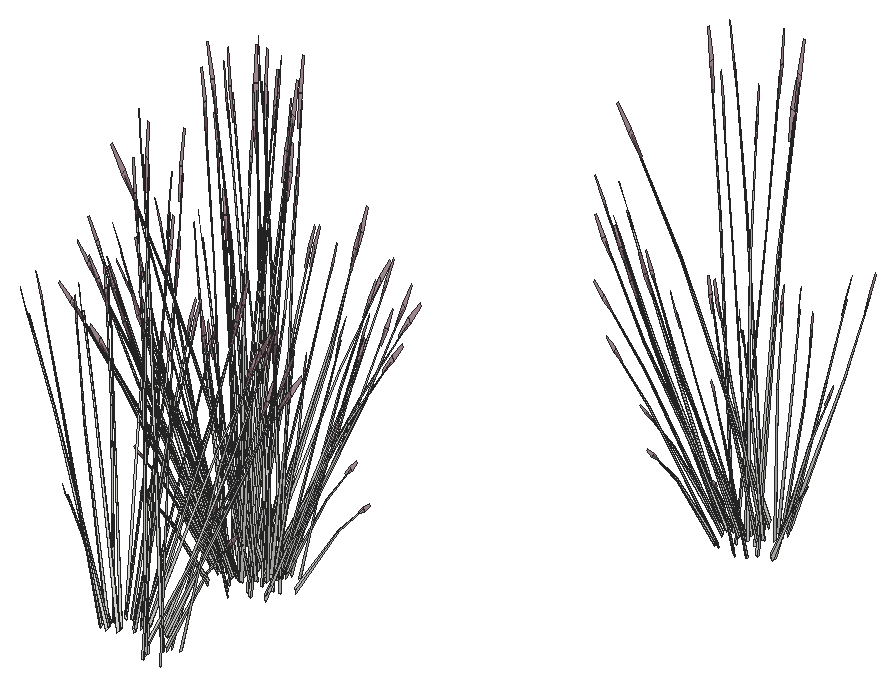
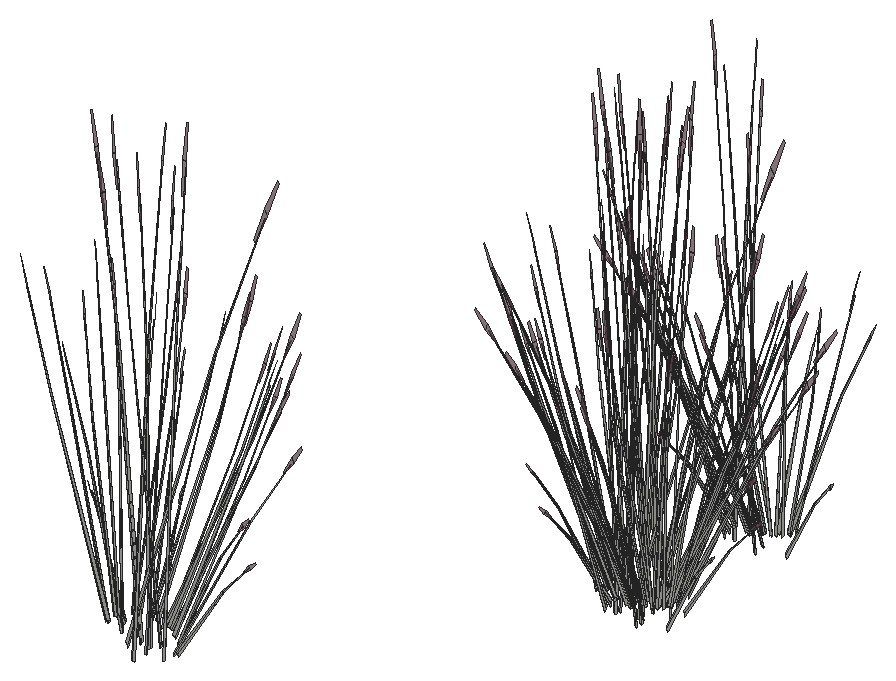
# SketchUp Ruby script. Lengths in inches.
U = 1.inch
M = Sketchup.active_model
def pt(a) = Geom::Point3d.new(a.map { |v| v * U })
def face(e, loops, mat)
  f = e.add_face(loops[0].map { |a| pt(a) })
  loops[1..].each { |l| e.add_face(l.map { |a| pt(a) }).erase! }
  f.material = f.back_material = mat if mat
  f
end
# faces: each face lists its corners as indices into pts; further lists are holes
def faces(e, pts, list, mat = nil) = list.each { |f| face(e, (f[0].is_a?(Array) ? f : [f]).map { |l| l.map { |i| pts[i] } }, mat) }
# xy, xz, yz: faces in a plane at the given z, y or x. An outline is a flat list of corners, or four numbers for a rectangle; further outlines are holes
def ring(l) = l.size == 4 ? [[l[0], l[1]], [l[2], l[1]], [l[2], l[3]], [l[0], l[3]]] : l.each_slice(2).to_a
def flat(e, list, mat, &to3) = list.each { |f| face(e, (f[0].is_a?(Array) ? f : [f]).map { |l| ring(l).map { |u, v| to3.(u, v) } }, mat) }
def xy(e, z, list, mat = nil) = flat(e, list, mat) { |x, y| [x, y, z] }
def xz(e, y, list, mat = nil) = flat(e, list, mat) { |x, z| [x, y, z] }
def yz(e, x, list, mat = nil) = flat(e, list, mat) { |y, z| [x, y, z] }
def lines(e, pts, list) = list.each { |a, b| e.add_line(pt(pts[a]), pt(pts[b])) }
# prism: a flat outline (further loops are holes) pulled along v
def prism(e, loops, v, mat = nil)
  f = face(e, loops, mat); d = Geom::Vector3d.new(v.map { |x| x * U })
  f.pushpull(f.normal.samedirection?(d) ? d.length : -d.length)
end
def box(e, o, s, mat = nil) = prism(e, [[o, [o[0] + s[0], o[1], o[2]], [o[0] + s[0], o[1] + s[1], o[2]], [o[0], o[1] + s[1], o[2]]]], [0, 0, s[2]], mat)
def at(x, y, z, deg = 0) = Geom::Transformation.translation(pt([x, y, z])) * Geom::Transformation.rotation(ORIGIN, Z_AXIS, deg.degrees)
def axes(o, x, y, z) = Geom::Transformation.new([*x, 0, *y, 0, *z, 0, *pt(o).to_a, 1])
def part(name) = M.definitions.add(name)
# library, detail: a bought-in or finely detailed component or shape, given as its bounding box
def library(name, o, s) = part(name).tap { |d| box(d.entities, o, s) }
def detail(e, o, s) = box(e.add_group.entities, o, s)
def put(e, d, t, mat = nil) = e.add_instance(d, t).tap { |i| i.material = mat if mat }
def group(e, t, mat = nil) = e.add_group.tap { |g| g.transformation = t; g.material = mat if mat }.entities
root = M.entities
M.materials.add("LightPink_Translucent").color = [144, 107, 117]
M.materials["LightPink_Translucent"].alpha = 0.75
c1 = part("blade")
p = [[2.15,0.21,22],[0,0.17,0],[0.09,0.45,0],[2.18,0.31,22],[2.29,0.31,22],[0.38,0.45,0],
  [2.48,0.24,33],[2.49,0.24,33],[2.48,0.22,33]]
faces(c1.entities,p,[[0,1,2,3],[4,5,2,3],[6,3,4,7],[8,0,3,6]])
c2 = part("seeds")
p = [[0.3,-0.1,1.38],[-0.01,-0.03,1.59],[-0.01,-0.03,0.03],[0.14,-0.07,-0.07],[0.29,-0.03,3],[0.15,0.01,3.11]]
faces(c2.entities,p,[[0,1,2,3],[1,0,4,5]],"LightPink_Translucent")
c3 = part("blade with seeds")
put(c3.entities,c1,at(0,0,0))
put(c3.entities,c2,axes([2.4,0.25,30.99],[1.5799,-0.05474,1.17369],[-0.12525,1.92788,0.29478],[-0.07173,-0.02425,1.56792]))
put(root,c3,axes([672.75,276.61,512.26],[0.31565,-0.51449,0.37133],[0.65588,0.24761,-0.17871],[0,0.1186,1.19224]))
put(root,c3,axes([668.89,276.66,513.89],[-0.17625,0.51936,-0.42412],[-0.60429,-0.17802,-0.32852],[-0.2433,0.04762,0.81151]))
put(root,c3,axes([675.33,278.46,513.26],[-0.12452,-0.47997,-0.02898],[0.58854,-0.11034,-0.1314],[0.1229,0.03043,0.43341]))
put(root,c3,axes([674.4,276.89,512.06],[0,-0.57097,0.4121],[0.72788,0,0],[0,0.13004,1.30728]))
put(root,c3,axes([672.58,277.32,512.26],[0.70648,-0.03525,0.37133],[0.06389,0.58508,-0.17871],[-0.12647,0.0593,1.19224]))
put(root,c3,axes([668.875,276.93,513.22],[0.22574,-0.12077,1.42242],[0.19004,0.55807,0.11501],[-0.35439,0.12613,0.60807]))
put(root,c3,axes([673.83,278.16,514.13],[0.65035,0.01375,-0.58968],[-0.04368,0.5789,0.07116],[0.27552,0.06109,0.83415]))
put(root,c3,axes([673.1,278.63,512.06],[0.60889,-0.28548,0.4121],[0.36394,0.51192,0],[-0.13868,0.06502,1.30728]))
put(root,c3,axes([667.7,278.88,512.3],[0.27113,-0.25877,0.95334],[0.10699,0.40966,0.70045],[-0.19594,0.07335,0.20998]))
put(root,c3,axes([674.23,278.4,513.76],[0.37017,0.35748,-0.29394],[-0.42268,0.3384,0.37948],[0.21476,0.05149,0.72609]))
put(root,c3,axes([668.72,277.76,513.76],[-0.56631,0.0816,-0.29394],[-0.14954,-0.46647,0.37948],[-0.16229,0.12529,0.72609]))
put(root,c3,axes([672.9,277.49,513.22],[-0.24166,-0.09837,1.42242],[0.50011,-0.41269,0.11501],[0.3117,0.18617,0.60807]))
put(root,c3,axes([673.79,278.61,512.3],[-0.36631,-0.16417,0.95334],[0.47299,-0.16681,0.70045],[0.12758,0.1413,0.20998]))
put(root,c3,axes([669.7,277.3,513.22],[0.1625,-0.17544,1.42242],[0.41029,0.47354,0.11501],[-0.28141,0.21565,0.60807]))
put(root,c3,axes([669.1875,277.82,513.89],[0.16713,0.52135,-0.42412],[-0.63294,0.0912,-0.32852],[-0.18138,0.14003,0.81151]))
put(root,c3,axes([672.9,276.76,512.36],[-0.01777,-0.53759,1.17256],[0.80434,0.13935,0.49647],[-0.19024,0.29416,1.1068]))
put(root,c3,axes([672.96,278.83,513.89],[0.64198,-0.13573,-0.42412],[0.1123,0.514,-0.32852],[0.17243,0.1473,0.81151]))
put(root,c3,axes([673.85,279.35,512.21],[-0.4172,-0.01791,0.872],[0.27552,-0.38032,0.48145],[0.16481,0.13512,0.68401]))
put(root,c3,axes([669.58,277.74,513.22],[0.12114,-0.19625,1.42242],[0.50818,0.40613,0.11501],[-0.22925,0.25313,0.60807]))
put(root,c3,axes([669.72,278.84,513.76],[-0.4402,0.30062,-0.29394],[-0.41671,-0.34326,0.37948],[-0.0634,0.1744,0.72609]))
put(root,c3,axes([670,280.01,512.3],[-0.01684,-0.3395,0.95334],[0.42072,0.24214,0.70045],[-0.08274,0.16182,0.20998]))
put(root,c3,axes([670.16,278.7,514.15],[0.46573,0.38364,-0.47077],[-0.49199,0.33598,-0.36465],[-0.07086,0.19492,0.90078]))
put(root,c3,axes([671.54,279.07,513.89],[0.63954,0.14313,-0.42412],[-0.21921,0.49074,-0.32852],[0.05864,0.19758,0.81151]))
put(root,c3,axes([671.9,278.06,513.22],[-0.14872,-0.18332,1.42242],[0.6872,-0.15433,0.11501],[0.15531,0.28779,0.60807]))
put(root,c3,axes([671.25,279.375,513.76],[-0.19614,0.43908,-0.29394],[-0.57222,-0.12807,0.37948],[0.05247,0.17678,0.72609]))
put(root,c3,axes([670.01,278.52,514.43],[-0.01693,0.52814,-0.65454],[-0.71285,-0.03547,0.07899],[-0.07523,0.22375,0.92591]))
put(root,c3,axes([670.6875,278.15,513.22],[-0.01592,-0.21915,1.42242],[0.69015,0.14538,0.11501],[-0.04269,0.3123,0.60807]))
put(root,c3,axes([671.3,278.98,514.13],[0.31051,0.46426,-0.58968],[-0.63919,0.25873,0.07116],[0.07261,0.22432,0.83415]))
put(root,c3,axes([669.77,279.27,512.79],[0.01429,-0.29475,1.28107],[0.64291,0.15569,0.17703],[-0.0557,0.31414,0.60492]))
put(root,c3,axes([670.27,289.8,513.22],[0.14872,0.18332,1.42242],[-0.6872,0.15433,0.11501],[-0.15531,-0.28779,0.60807]))
put(root,c3,axes([672.1,289.94,514.13],[-0.31051,-0.46426,-0.58968],[0.63919,-0.25873,0.07116],[-0.07261,-0.22432,0.83415]))
put(root,c3,axes([673.39,290.39,514.13],[0.01693,-0.52814,-0.58968],[0.71285,0.03547,0.07116],[0.07523,-0.22375,0.83415]))
put(root,c3,axes([672.16,289.55,513.76],[0.19614,-0.43908,-0.29394],[0.57222,0.12807,0.37948],[-0.05247,-0.17678,0.72609]))
put(root,c3,axes([672.59,290.13,513.22],[-0.12114,0.19625,1.42242],[-0.50818,-0.40613,0.11501],[0.22925,-0.25313,0.60807]))
put(root,c3,axes([671.87,289.85,513.89],[-0.63954,-0.14313,-0.42412],[0.21921,-0.49074,-0.32852],[-0.05864,-0.19758,0.81151]))
put(root,c3,axes([672.26,288.62,512.3],[0.08346,0.33295,0.95334],[-0.46298,-0.1844,0.70045],[0.04982,-0.17048,0.20998]))
put(root,c3,axes([673.25,290.22,513.89],[-0.46573,-0.38364,-0.42412],[0.49199,-0.33598,-0.32852],[0.07086,-0.19492,0.81151]))
put(root,c3,axes([673.69,290.08,513.76],[0.4402,-0.30062,-0.29394],[0.41671,0.34326,0.37948],[0.0634,-0.1744,0.72609]))
put(root,c3,axes([669.88,289.02,512.3],[0.33937,0.19872,0.95334],[-0.49424,0.11946,0.70045],[-0.10575,-0.15273,0.20998]))
put(root,c3,axes([670.7,290.07,514.13],[-0.55475,-0.27598,-0.58968],[0.39425,-0.48361,0.07116],[-0.20099,-0.16478,0.83415]))
put(root,c3,axes([670.51,289.71,513.76],[-0.10048,-0.4599,-0.29394],[0.5744,-0.12144,0.37948],[-0.15428,-0.13179,0.72609]))
put(root,c3,axes([669.27,290.375,513.22],[0.24166,0.09837,1.42242],[-0.50011,0.41269,0.11501],[-0.3117,-0.18617,0.60807]))
put(root,c3,axes([670.44,290.09,513.89],[-0.64198,0.13573,-0.42412],[-0.1123,-0.514,-0.32852],[-0.17243,-0.1473,0.81151]))
put(root,c3,axes([674.23,291.3125,514.13],[0.33983,-0.45051,-0.58968],[0.59551,0.32017,0.07116],[0.20291,-0.16322,0.83415]))
put(root,c3,axes([674.21,291.1,513.89],[-0.16713,-0.52135,-0.42412],[0.63294,-0.0912,-0.32852],[0.18138,-0.14003,0.81151]))
put(root,c3,axes([672.03,293.19,512.76],[0.56221,0.23024,1.25546],[-0.55078,0.49601,0.49647],[-0.2467,-0.29398,1.05249]))
put(root,c3,axes([674.99,290.07,512.3],[-0.2167,0.29065,0.95334],[-0.18626,-0.3905,0.70045],[0.17898,-0.09785,0.20998]))
put(root,c3,axes([674.68,291.16,513.76],[0.56631,-0.0816,-0.29394],[0.14954,0.46647,0.37948],[0.16229,-0.12529,0.72609]))
put(root,c3,axes([669.18,290.52,513.76],[-0.37017,-0.35748,-0.29394],[0.42268,-0.3384,0.37948],[-0.21476,-0.05149,0.72609]))
put(root,c3,axes([669.57,290.75,514.13],[-0.65035,-0.01375,-0.58968],[0.04368,-0.5789,0.07116],[-0.27552,-0.06109,0.83415]))
put(root,c3,axes([669.35,290.87,513.89],[-0.47241,0.37822,-0.42412],[-0.41372,-0.39954,-0.32852],[-0.24002,-0.05755,0.81151]))
put(root,c3,axes([668.29,291.37,512.3],[0.41536,-0.04086,0.95334],[-0.26347,0.35999,0.70045],[-0.20525,-0.054,0.20998]))
put(root,c3,axes([671.22,291.71,512.26],[-0.70648,0.03525,0.37133],[-0.06389,-0.58508,-0.17871],[0.12647,-0.0593,1.19224]))
put(root,c3,axes([669.4,292.13,512.06],[0,0.57097,0.4121],[-0.72788,0,0],[0,-0.13004,1.30728]))
put(root,c3,axes([674.51,292.26,513.89],[0.17625,-0.51936,-0.42412],[0.60429,0.17802,-0.32852],[0.2433,-0.04762,0.81151]))
put(root,c3,axes([668.76,291.28,513.22],[0.26985,-0.01293,1.42242],[-0.17902,0.56047,0.11501],[-0.38456,-0.03467,0.60807]))
put(root,c3,axes([671.06,292.42,512.26],[-0.31565,0.51449,0.37133],[-0.65588,-0.24761,-0.17871],[0,-0.1186,1.19224]))
put(root,c3,axes([673.2,290.44,512.06],[-0.60889,-0.28548,0.4121],[0.36394,-0.51192,0],[0.13868,0.06502,1.30728]))
put(root,c3,axes([674.39,292.45,514.13],[0.57168,-0.25217,-0.58968],[0.3186,0.51908,0.07116],[0.27622,-0.05897,0.83415]))
put(root,c3,axes([670.89,290.7,512.05],[-0.18794,0.56744,0.14643],[-0.68774,-0.16058,0.29122],[0.1188,-0.00276,1.33138]))
put(root,c3,axes([672.07,291.47,512.26],[-0.39083,-0.47924,0.37133],[0.59199,-0.33747,-0.17871],[0.12647,0.0593,1.19224]))
put(root,c3,axes([670.83,293.63,512.05],[0.6991,-0.15154,0.14643],[0.17263,0.56398,0.29122],[-0.06235,-0.08217,1.33138]))
put(root,c3,axes([674.88,292.5,513.76],[0.54068,0.15928,-0.29394],[-0.1577,0.46469,0.37948],[0.21769,-0.04261,0.72609]))
put(root,c3,axes([668.52,291.76,513.76],[-0.54068,-0.15928,-0.29394],[0.1577,-0.46469,0.37948],[-0.21769,0.04261,0.72609]))
put(root,c3,axes([672.97,290.73,512.05],[-0.6991,0.15154,0.14643],[-0.17263,-0.56398,0.29122],[0.06235,0.08217,1.33138]))
put(root,c3,axes([673.41,291.92,513.22],[-0.26985,0.01293,1.42242],[0.17902,-0.56047,0.11501],[0.38456,0.03467,0.60807]))
put(root,c3,axes([672.91,293.66,512.05],[0.18794,-0.56744,0.14643],[0.68774,0.16058,0.29122],[-0.1188,0.00276,1.33138]))
put(root,c3,axes([670.17,291.68,512.77],[0.18493,-0.0826,1.46963],[0.06377,0.5767,0.11501],[-0.40056,0.07652,0.52526]))
put(root,c3,axes([673.98,292.21,512.05],[-0.51116,-0.4159,0.14643],[0.51512,-0.4034,0.29122],[-0.05645,0.08494,1.33138]))
put(root,c3,axes([676.03,292.59,512.3],[-0.40197,0.09426,0.95334],[0.18921,-0.38956,0.70045],[0.21325,0.02666,0.20998]))
put(root,c3,axes([670.6,293.92,512.06],[0.60889,0.28548,0.4121],[-0.36394,0.51192,0],[-0.13868,-0.06502,1.30728]))
put(root,c3,axes([672.75,291.94,512.26],[0.31565,-0.51449,0.37133],[0.65588,0.24761,-0.17871],[0,0.1186,1.19224]))
put(root,c3,axes([668.89,291.99,513.89],[-0.17625,0.51936,-0.42412],[-0.60429,-0.17802,-0.32852],[-0.2433,0.04762,0.81151]))
put(root,c3,axes([675.33,293.79,513.26],[-0.12452,-0.47997,-0.02898],[0.58854,-0.11034,-0.1314],[0.1229,0.03043,0.43341]))
put(root,c3,axes([674.4,292.23,512.06],[0,-0.57097,0.4121],[0.72788,0,0],[0,0.13004,1.30728]))
put(root,c3,axes([672.58,292.65,512.26],[0.70648,-0.03525,0.37133],[0.06389,0.58508,-0.17871],[-0.12647,0.0593,1.19224]))
put(root,c3,axes([668.875,292.26,513.22],[0.22574,-0.12077,1.42242],[0.19004,0.55807,0.11501],[-0.35439,0.12613,0.60807]))
put(root,c3,axes([673.83,293.5,514.13],[0.65035,0.01375,-0.58968],[-0.04368,0.5789,0.07116],[0.27552,0.06109,0.83415]))
put(root,c3,axes([673.1,293.96,512.06],[0.60889,-0.28548,0.4121],[0.36394,0.51192,0],[-0.13868,0.06502,1.30728]))
put(root,c3,axes([667.7,294.22,512.3],[0.27113,-0.25877,0.95334],[0.10699,0.40966,0.70045],[-0.19594,0.07335,0.20998]))
put(root,c3,axes([674.23,293.74,513.76],[0.37017,0.35748,-0.29394],[-0.42268,0.3384,0.37948],[0.21476,0.05149,0.72609]))
put(root,c3,axes([668.72,293.1,513.76],[-0.56631,0.0816,-0.29394],[-0.14954,-0.46647,0.37948],[-0.16229,0.12529,0.72609]))
put(root,c3,axes([672.9,292.82,513.22],[-0.24166,-0.09837,1.42242],[0.50011,-0.41269,0.11501],[0.3117,0.18617,0.60807]))
put(root,c3,axes([673.79,293.94,512.3],[-0.36631,-0.16417,0.95334],[0.47299,-0.16681,0.70045],[0.12758,0.1413,0.20998]))
put(root,c3,axes([669.7,292.64,513.22],[0.1625,-0.17544,1.42242],[0.41029,0.47354,0.11501],[-0.28141,0.21565,0.60807]))
put(root,c3,axes([669.1875,293.15,513.89],[0.16713,0.52135,-0.42412],[-0.63294,0.0912,-0.32852],[-0.18138,0.14003,0.81151]))
put(root,c3,axes([672.9,292.09,512.36],[-0.01777,-0.53759,1.17256],[0.80434,0.13935,0.49647],[-0.19024,0.29416,1.1068]))
put(root,c3,axes([672.96,294.17,513.89],[0.64198,-0.13573,-0.42412],[0.1123,0.514,-0.32852],[0.17243,0.1473,0.81151]))
put(root,c3,axes([673.85,294.6875,512.21],[-0.4172,-0.01791,0.872],[0.27552,-0.38032,0.48145],[0.16481,0.13512,0.68401]))
put(root,c3,axes([669.58,293.07,513.22],[0.12114,-0.19625,1.42242],[0.50818,0.40613,0.11501],[-0.22925,0.25313,0.60807]))
put(root,c3,axes([669.72,294.18,513.76],[-0.4402,0.30062,-0.29394],[-0.41671,-0.34326,0.37948],[-0.0634,0.1744,0.72609]))
put(root,c3,axes([670,295.34,512.3],[-0.01684,-0.3395,0.95334],[0.42072,0.24214,0.70045],[-0.08274,0.16182,0.20998]))
put(root,c3,axes([670.16,294.03,514.15],[0.46573,0.38364,-0.47077],[-0.49199,0.33598,-0.36465],[-0.07086,0.19492,0.90078]))
put(root,c3,axes([671.54,294.41,513.89],[0.63954,0.14313,-0.42412],[-0.21921,0.49074,-0.32852],[0.05864,0.19758,0.81151]))
put(root,c3,axes([671.9,293.39,513.22],[-0.14872,-0.18332,1.42242],[0.6872,-0.15433,0.11501],[0.15531,0.28779,0.60807]))
put(root,c3,axes([671.25,294.71,513.76],[-0.19614,0.43908,-0.29394],[-0.57222,-0.12807,0.37948],[0.05247,0.17678,0.72609]))
put(root,c3,axes([670.01,293.86,514.43],[-0.01693,0.52814,-0.65454],[-0.71285,-0.03547,0.07899],[-0.07523,0.22375,0.92591]))
put(root,c3,axes([670.6875,293.48,513.22],[-0.01592,-0.21915,1.42242],[0.69015,0.14538,0.11501],[-0.04269,0.3123,0.60807]))
put(root,c3,axes([671.3,294.3125,514.13],[0.31051,0.46426,-0.58968],[-0.63919,0.25873,0.07116],[0.07261,0.22432,0.83415]))
put(root,c3,axes([669.77,294.6,512.79],[0.01429,-0.29475,1.28107],[0.64291,0.15569,0.17703],[-0.0557,0.31414,0.60492]))
put(root,c3,axes([700.55,320.23,512.15],[-0.18493,0.11557,1.18691],[-0.55384,-0.20228,-0.25526],[0.10266,-0.25157,0.50747]))
put(root,c3,axes([699.7,320.63,514.13],[-0.31051,-0.46426,-0.58968],[0.63919,-0.25873,0.07116],[-0.07261,-0.22432,0.83415]))
put(root,c3,axes([697.68,320.01,512.15],[-0.0394,0.18678,1.18691],[-0.57594,0.15636,-0.25526],[-0.13463,-0.24142,0.50747]))
put(root,c3,axes([701,321.09,514.13],[0.01693,-0.52814,-0.58968],[0.71285,0.03547,0.07116],[0.07523,-0.22375,0.83415]))
put(root,c3,axes([699.76,320.24,513.76],[0.19614,-0.43908,-0.29394],[0.57222,0.12807,0.37948],[-0.05247,-0.17678,0.72609]))
put(root,c3,axes([699.47,320.54,513.89],[-0.63954,-0.14313,-0.42412],[0.21921,-0.49074,-0.32852],[-0.05864,-0.19758,0.81151]))
put(root,c3,axes([699.87,319.31,512.3],[0.08346,0.33295,0.95334],[-0.46298,-0.1844,0.70045],[0.04982,-0.17048,0.20998]))
put(root,c3,axes([700.85,320.91,513.89],[-0.46573,-0.38364,-0.42412],[0.49199,-0.33598,-0.32852],[0.07086,-0.19492,0.81151]))
put(root,c3,axes([701.29,320.77,513.76],[0.4402,-0.30062,-0.29394],[0.41671,0.34326,0.37948],[0.0634,-0.1744,0.72609]))
put(root,c3,axes([697.49,319.71,512.3],[0.33937,0.19872,0.95334],[-0.49424,0.11946,0.70045],[-0.10575,-0.15273,0.20998]))
put(root,c3,axes([698.3,320.76,514.13],[-0.55475,-0.27598,-0.58968],[0.39425,-0.48361,0.07116],[-0.20099,-0.16478,0.83415]))
put(root,c3,axes([698.11,320.4,513.76],[-0.10048,-0.4599,-0.29394],[0.5744,-0.12144,0.37948],[-0.15428,-0.13179,0.72609]))
put(root,c3,axes([698.05,320.78,513.89],[-0.64198,0.13573,-0.42412],[-0.1123,-0.514,-0.32852],[-0.17243,-0.1473,0.81151]))
put(root,c3,axes([701.84,322,514.13],[0.33983,-0.45051,-0.58968],[0.59551,0.32017,0.07116],[0.20291,-0.16322,0.83415]))
put(root,c3,axes([701.82,321.79,513.89],[-0.16713,-0.52135,-0.42412],[0.63294,-0.0912,-0.32852],[0.18138,-0.14003,0.81151]))
put(root,c3,axes([699.63,323.89,512.76],[0.56221,0.23024,1.25546],[-0.55078,0.49601,0.49647],[-0.2467,-0.29398,1.05249]))
put(root,c3,axes([702.33,321.59,512.15],[-0.23242,-0.01691,1.18691],[-0.23811,-0.45367,-0.25526],[0.28553,-0.12834,0.50747]))
put(root,c3,axes([702.6,320.76,512.3],[-0.2167,0.29065,0.95334],[-0.18626,-0.3905,0.70045],[0.17898,-0.09785,0.20998]))
put(root,c3,axes([702.29,321.85,513.76],[0.56631,-0.0816,-0.29394],[0.14954,0.46647,0.37948],[0.16229,-0.12529,0.72609]))
put(root,c3,axes([696.78,321.21,513.76],[-0.37017,-0.35748,-0.29394],[0.42268,-0.3384,0.37948],[-0.21476,-0.05149,0.72609]))
put(root,c3,axes([696.65,321.59,512.15],[0.12702,0.15896,1.18691],[-0.2927,0.4321,-0.25526],[-0.30054,-0.10328,0.50747]))
put(root,c3,axes([697.17,321.45,514.13],[-0.65035,-0.01375,-0.58968],[0.04368,-0.5789,0.07116],[-0.27552,-0.06109,0.83415]))
put(root,c3,axes([696.96,321.5625,513.89],[-0.47241,0.37822,-0.42412],[-0.41372,-0.39954,-0.32852],[-0.24002,-0.05755,0.81151]))
put(root,c3,axes([695.89,322.06,512.3],[0.41536,-0.04086,0.95334],[-0.26347,0.35999,0.70045],[-0.20525,-0.054,0.20998]))
put(root,c3,axes([698.83,322.4,512.26],[-0.70648,0.03525,0.37133],[-0.06389,-0.58508,-0.17871],[0.12647,-0.0593,1.19224]))
put(root,c3,axes([697.01,322.82,512.06],[0,0.57097,0.4121],[-0.72788,0,0],[0,-0.13004,1.30728]))
put(root,c3,axes([702.11,322.95,513.89],[0.17625,-0.51936,-0.42412],[0.60429,0.17802,-0.32852],[0.2433,-0.04762,0.81151]))
put(root,c3,axes([698.66,323.11,512.26],[-0.31565,0.51449,0.37133],[-0.65588,-0.24761,-0.17871],[0,-0.1186,1.19224]))
put(root,c3,axes([700.81,321.14,512.06],[-0.60889,-0.28548,0.4121],[0.36394,-0.51192,0],[0.13868,0.06502,1.30728]))
put(root,c3,axes([702,323.14,514.13],[0.57168,-0.25217,-0.58968],[0.3186,0.51908,0.07116],[0.27622,-0.05897,0.83415]))
put(root,c3,axes([698.5,321.39,512.05],[-0.18794,0.56744,0.14643],[-0.68774,-0.16058,0.29122],[0.1188,-0.00276,1.33138]))
put(root,c3,axes([699.67,322.16,512.26],[-0.39083,-0.47924,0.37133],[0.59199,-0.33747,-0.17871],[0.12647,0.0593,1.19224]))
put(root,c3,axes([698.43,324.32,512.05],[0.6991,-0.15154,0.14643],[0.17263,0.56398,0.29122],[-0.06235,-0.08217,1.33138]))
